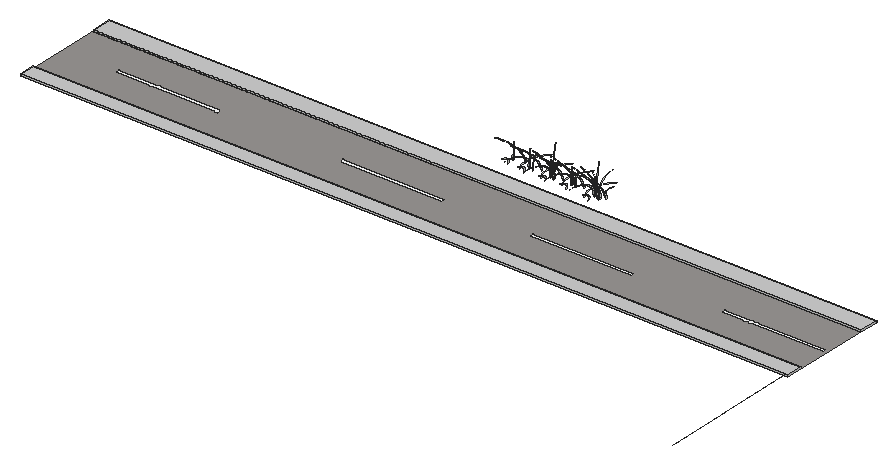
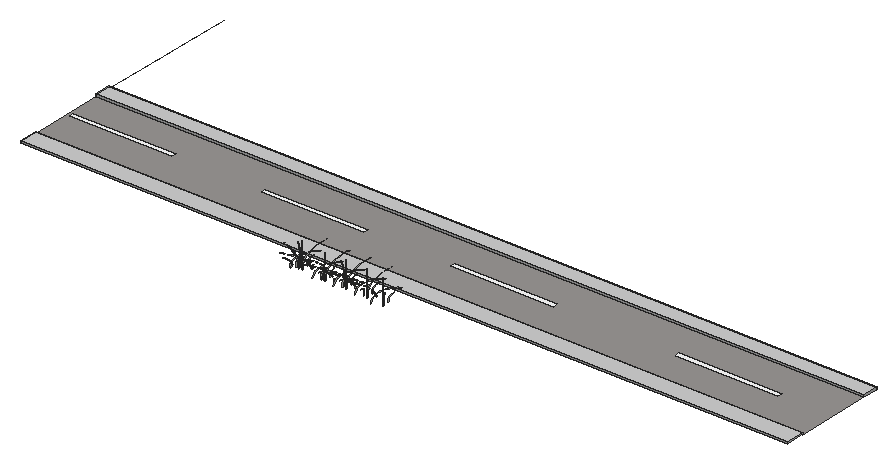
# SketchUp Ruby script. Lengths in inches.
U = 1.inch
M = Sketchup.active_model
def pt(a) = Geom::Point3d.new(a.map { |v| v * U })
def face(e, loops, mat)
  f = e.add_face(loops[0].map { |a| pt(a) })
  loops[1..].each { |l| e.add_face(l.map { |a| pt(a) }).erase! }
  f.material = f.back_material = mat if mat
  f
end
# faces: each face lists its corners as indices into pts; further lists are holes
def faces(e, pts, list, mat = nil) = list.each { |f| face(e, (f[0].is_a?(Array) ? f : [f]).map { |l| l.map { |i| pts[i] } }, mat) }
# xy, xz, yz: faces in a plane at the given z, y or x. An outline is a flat list of corners, or four numbers for a rectangle; further outlines are holes
def ring(l) = l.size == 4 ? [[l[0], l[1]], [l[2], l[1]], [l[2], l[3]], [l[0], l[3]]] : l.each_slice(2).to_a
def flat(e, list, mat, &to3) = list.each { |f| face(e, (f[0].is_a?(Array) ? f : [f]).map { |l| ring(l).map { |u, v| to3.(u, v) } }, mat) }
def xy(e, z, list, mat = nil) = flat(e, list, mat) { |x, y| [x, y, z] }
def xz(e, y, list, mat = nil) = flat(e, list, mat) { |x, z| [x, y, z] }
def yz(e, x, list, mat = nil) = flat(e, list, mat) { |y, z| [x, y, z] }
def lines(e, pts, list) = list.each { |a, b| e.add_line(pt(pts[a]), pt(pts[b])) }
# prism: a flat outline (further loops are holes) pulled along v
def prism(e, loops, v, mat = nil)
  f = face(e, loops, mat); d = Geom::Vector3d.new(v.map { |x| x * U })
  f.pushpull(f.normal.samedirection?(d) ? d.length : -d.length)
end
def box(e, o, s, mat = nil) = prism(e, [[o, [o[0] + s[0], o[1], o[2]], [o[0] + s[0], o[1] + s[1], o[2]], [o[0], o[1] + s[1], o[2]]]], [0, 0, s[2]], mat)
def at(x, y, z, deg = 0) = Geom::Transformation.translation(pt([x, y, z])) * Geom::Transformation.rotation(ORIGIN, Z_AXIS, deg.degrees)
def axes(o, x, y, z) = Geom::Transformation.new([*x, 0, *y, 0, *z, 0, *pt(o).to_a, 1])
def part(name) = M.definitions.add(name)
# library, detail: a bought-in or finely detailed component or shape, given as its bounding box
def library(name, o, s) = part(name).tap { |d| box(d.entities, o, s) }
def detail(e, o, s) = box(e.add_group.entities, o, s)
def put(e, d, t, mat = nil) = e.add_instance(d, t).tap { |i| i.material = mat if mat }
def group(e, t, mat = nil) = e.add_group.tap { |g| g.transformation = t; g.material = mat if mat }.entities
root = M.entities
M.materials.add("[Cladding_Siding_White]").color = [207, 207, 207]
M.materials.add("[Color_000]").color = [255, 255, 255]
M.materials.add("[Concrete_Aggregate_Smoke]").color = [154, 150, 148]
c1 = part("Untitled\#1")
xy(c1.entities,0,[[0,0,18.1875,211.875]],"[Cladding_Siding_White]")
xy(c1.entities,0,[[52.26,14.82,56.57,43.13],[53.72,77.12,58.03,105.43],[54.1,129.57,58.41,157.89],[54.67,182.79,58.98,211.1]],"[Color_000]")
xy(c1.entities,0,[[[18.1875,-0.0625,89.875,211.875],[52.26,14.82,56.57,43.13],[53.72,77.12,58.03,105.43],[54.1,129.57,58.41,157.89],[54.67,182.79,58.98,211.1]]],"[Concrete_Aggregate_Smoke]")
xy(c1.entities,1.625,[[0,0,18.1875,211.875]],"[Cladding_Siding_White]")
xy(c1.entities,1.9375,[[89.875,-0.0625,105,211.9375]],"[Cladding_Siding_White]")
xz(c1.entities,-0.0625,[[89.875,0,105,1.9375]],"[Cladding_Siding_White]")
xz(c1.entities,0,[[0,0,18.1875,1.625]],"[Cladding_Siding_White]")
xz(c1.entities,211.875,[[0,0,18.1875,1.625]],"[Cladding_Siding_White]")
xz(c1.entities,211.9375,[[89.875,0,105,1.9375]],"[Cladding_Siding_White]")
yz(c1.entities,0,[[0,0,211.875,1.625]],"[Cladding_Siding_White]")
yz(c1.entities,18.1875,[[0,0,211.875,1.625]],"[Cladding_Siding_White]")
yz(c1.entities,89.875,[[-0.0625,0,211.875,1.9375],[211.875,0,211.9375,1.9375]],"[Cladding_Siding_White]")
yz(c1.entities,105,[[-0.0625,0,211.9375,1.9375]],"[Cladding_Siding_White]")
p = [[799.67,134.13,1.9375],[799.67,0,0]]
lines(root,p,[[0,1]])
put(root,c1,axes([75.64,239.13,0],[0,-1,0],[3.42659,0,0],[0,0,1]))
g1 = group(root,at(519.48,258.51,0))
p = [[-0.1,-0.92,0],[-0.05,-0.41,0],[0,0,2.0625],[-0.02,-0.17,4.13],[-0.1,-0.9,6.16],[-0.24,-2.1875,8.1],
  [-0.44,-3.99,9.91],[-0.69,-6.27,11.52],[-0.99,-8.97,12.92],[-1.33,-12.02,14.05],[-1.69,-15.34,14.9],[-2.08,-18.86,15.45],
  [-2.48,-22.49,15.67],[-2.88,-26.13,15.5625],[-2.49,-22.56,15.58],[-2.1,-19.02,15.29],[-1.72,-15.6,14.71],[-1.37,-12.38,13.83],
  [-1.04,-9.43,12.68],[-0.75,-6.81,11.3],[-0.51,-4.6,9.7],[-0.3125,-2.84,7.9375],[-0.17,-1.5625,6.04],[-0.09,-0.81,4.05],
  [-0.07,-0.59,2.02]]
faces(g1,p,[[0,1,2,3,4,5,6,7,8,9,10,11,12,13,14,15,16,17,18,19,20,21,22,23,24]])
g2 = group(root,at(519.48,258.51,0))
p = [[-0.1,-0.92,0],[-0.05,-0.41,0],[0,0,2.0625],[-0.02,-0.17,4.13],[-0.1,-0.9,6.16],[-0.24,-2.1875,8.1],
  [-0.44,-3.99,9.91],[-0.69,-6.27,11.52],[-0.99,-8.97,12.92],[-1.33,-12.02,14.05],[-1.69,-15.34,14.9],[-2.08,-18.86,15.45],
  [-2.48,-22.49,15.67],[-2.88,-26.13,15.5625],[-2.49,-22.56,15.58],[-2.1,-19.02,15.29],[-1.72,-15.6,14.71],[-1.37,-12.38,13.83],
  [-1.04,-9.43,12.68],[-0.75,-6.81,11.3],[-0.51,-4.6,9.7],[-0.3125,-2.84,7.9375],[-0.17,-1.5625,6.04],[-0.09,-0.81,4.05],
  [-0.07,-0.59,2.02]]
faces(g2,p,[[0,1,2,3,4,5,6,7,8,9,10,11,12,13,14,15,16,17,18,19,20,21,22,23,24]])
g3 = group(root,at(476.43,260.84,0))
p = [[-0.1,-0.92,0],[-0.05,-0.41,0],[0,0,2.0625],[-0.02,-0.17,4.13],[-0.1,-0.9,6.16],[-0.24,-2.1875,8.1],
  [-0.44,-3.99,9.91],[-0.69,-6.27,11.52],[-0.99,-8.97,12.92],[-1.33,-12.02,14.05],[-1.69,-15.34,14.9],[-2.08,-18.86,15.45],
  [-2.48,-22.49,15.67],[-2.88,-26.13,15.5625],[-2.49,-22.56,15.58],[-2.1,-19.02,15.29],[-1.72,-15.6,14.71],[-1.37,-12.38,13.83],
  [-1.04,-9.43,12.68],[-0.75,-6.81,11.3],[-0.51,-4.6,9.7],[-0.3125,-2.84,7.9375],[-0.17,-1.5625,6.04],[-0.09,-0.81,4.05],
  [-0.07,-0.59,2.02]]
faces(g3,p,[[0,1,2,3,4,5,6,7,8,9,10,11,12,13,14,15,16,17,18,19,20,21,22,23,24]])
g4 = group(root,at(476.43,260.84,0))
p = [[-0.1,-0.92,0],[-0.05,-0.41,0],[0,0,2.0625],[-0.02,-0.17,4.13],[-0.1,-0.9,6.16],[-0.24,-2.1875,8.1],
  [-0.44,-3.99,9.91],[-0.69,-6.27,11.52],[-0.99,-8.97,12.92],[-1.33,-12.02,14.05],[-1.69,-15.34,14.9],[-2.08,-18.86,15.45],
  [-2.48,-22.49,15.67],[-2.88,-26.13,15.5625],[-2.49,-22.56,15.58],[-2.1,-19.02,15.29],[-1.72,-15.6,14.71],[-1.37,-12.38,13.83],
  [-1.04,-9.43,12.68],[-0.75,-6.81,11.3],[-0.51,-4.6,9.7],[-0.3125,-2.84,7.9375],[-0.17,-1.5625,6.04],[-0.09,-0.81,4.05],
  [-0.07,-0.59,2.02]]
faces(g4,p,[[0,1,2,3,4,5,6,7,8,9,10,11,12,13,14,15,16,17,18,19,20,21,22,23,24]])
g5 = group(root,at(520.28,251.6,0))
p = [[-0.91,-7.12,6.7],[-0.75,-5.82,6.27],[-0.6,-4.64,5.81],[-0.46,-3.6,5.31],[-0.35,-2.71,4.77],[-0.25,-1.97,4.21],
  [-0.18,-1.39,3.63],[-0.125,-0.98,3.03],[-0.09,-0.74,2.43],[-0.09,-0.67,1.8125],[-0.1,-0.77,1.2],[-0.13,-1.05,0.59],
  [-0.19,-1.49,0],[-0.12,-0.92,0],[-0.05,-0.42,0.6],[-0.01,-0.11,1.22],[0,0,1.84],[-0.01,-0.08,2.47],
  [-0.04,-0.35,3.09],[-0.1,-0.81,3.69],[-0.1875,-1.45,4.28],[-0.29,-2.27,4.84],[-0.42,-3.26,5.37],[-0.57,-4.41,5.86],
  [-0.73,-5.7,6.3]]
faces(g5,p,[[0,1,2,3,4,5,6,7,8,9,10,11,12,13,14,15,16,17,18,19,20,21,22,23,24]])
g6 = group(root,at(495.91,261.57,0))
p = [[-0.1,-0.92,0],[-0.05,-0.41,0],[0,0,2.0625],[-0.02,-0.17,4.13],[-0.1,-0.9,6.16],[-0.24,-2.1875,8.1],
  [-0.44,-3.99,9.91],[-0.69,-6.27,11.52],[-0.99,-8.97,12.92],[-1.33,-12.02,14.05],[-1.69,-15.34,14.9],[-2.08,-18.86,15.45],
  [-2.48,-22.49,15.67],[-2.88,-26.13,15.5625],[-2.49,-22.56,15.58],[-2.1,-19.02,15.29],[-1.72,-15.6,14.71],[-1.37,-12.38,13.83],
  [-1.04,-9.43,12.68],[-0.75,-6.81,11.3],[-0.51,-4.6,9.7],[-0.3125,-2.84,7.9375],[-0.17,-1.5625,6.04],[-0.09,-0.81,4.05],
  [-0.07,-0.59,2.02]]
faces(g6,p,[[0,1,2,3,4,5,6,7,8,9,10,11,12,13,14,15,16,17,18,19,20,21,22,23,24]])
g7 = group(root,at(495.91,261.57,0))
p = [[-0.1,-0.92,0],[-0.05,-0.41,0],[0,0,2.0625],[-0.02,-0.17,4.13],[-0.1,-0.9,6.16],[-0.24,-2.1875,8.1],
  [-0.44,-3.99,9.91],[-0.69,-6.27,11.52],[-0.99,-8.97,12.92],[-1.33,-12.02,14.05],[-1.69,-15.34,14.9],[-2.08,-18.86,15.45],
  [-2.48,-22.49,15.67],[-2.88,-26.13,15.5625],[-2.49,-22.56,15.58],[-2.1,-19.02,15.29],[-1.72,-15.6,14.71],[-1.37,-12.38,13.83],
  [-1.04,-9.43,12.68],[-0.75,-6.81,11.3],[-0.51,-4.6,9.7],[-0.3125,-2.84,7.9375],[-0.17,-1.5625,6.04],[-0.09,-0.81,4.05],
  [-0.07,-0.59,2.02]]
faces(g7,p,[[0,1,2,3,4,5,6,7,8,9,10,11,12,13,14,15,16,17,18,19,20,21,22,23,24]])
g8 = group(root,at(455.77,261.59,0))
p = [[-0.1,-0.92,0],[-0.05,-0.41,0],[0,0,2.0625],[-0.02,-0.17,4.13],[-0.1,-0.9,6.16],[-0.24,-2.1875,8.1],
  [-0.44,-3.99,9.91],[-0.69,-6.27,11.52],[-0.99,-8.97,12.92],[-1.33,-12.02,14.05],[-1.69,-15.34,14.9],[-2.08,-18.86,15.45],
  [-2.48,-22.49,15.67],[-2.88,-26.13,15.5625],[-2.49,-22.56,15.58],[-2.1,-19.02,15.29],[-1.72,-15.6,14.71],[-1.37,-12.38,13.83],
  [-1.04,-9.43,12.68],[-0.75,-6.81,11.3],[-0.51,-4.6,9.7],[-0.3125,-2.84,7.9375],[-0.17,-1.5625,6.04],[-0.09,-0.81,4.05],
  [-0.07,-0.59,2.02]]
faces(g8,p,[[0,1,2,3,4,5,6,7,8,9,10,11,12,13,14,15,16,17,18,19,20,21,22,23,24]])
g9 = group(root,at(455.77,261.59,0))
p = [[-0.1,-0.92,0],[-0.05,-0.41,0],[0,0,2.0625],[-0.02,-0.17,4.13],[-0.1,-0.9,6.16],[-0.24,-2.1875,8.1],
  [-0.44,-3.99,9.91],[-0.69,-6.27,11.52],[-0.99,-8.97,12.92],[-1.33,-12.02,14.05],[-1.69,-15.34,14.9],[-2.08,-18.86,15.45],
  [-2.48,-22.49,15.67],[-2.88,-26.13,15.5625],[-2.49,-22.56,15.58],[-2.1,-19.02,15.29],[-1.72,-15.6,14.71],[-1.37,-12.38,13.83],
  [-1.04,-9.43,12.68],[-0.75,-6.81,11.3],[-0.51,-4.6,9.7],[-0.3125,-2.84,7.9375],[-0.17,-1.5625,6.04],[-0.09,-0.81,4.05],
  [-0.07,-0.59,2.02]]
faces(g9,p,[[0,1,2,3,4,5,6,7,8,9,10,11,12,13,14,15,16,17,18,19,20,21,22,23,24]])
g10 = group(root,at(477.23,253.93,0))
p = [[-0.91,-7.12,6.7],[-0.75,-5.82,6.27],[-0.6,-4.64,5.81],[-0.46,-3.6,5.31],[-0.35,-2.71,4.77],[-0.25,-1.97,4.21],
  [-0.18,-1.39,3.63],[-0.125,-0.98,3.03],[-0.09,-0.74,2.43],[-0.09,-0.67,1.8125],[-0.1,-0.77,1.2],[-0.13,-1.05,0.59],
  [-0.19,-1.49,0],[-0.12,-0.92,0],[-0.05,-0.42,0.6],[-0.01,-0.11,1.22],[0,0,1.84],[-0.01,-0.08,2.47],
  [-0.04,-0.35,3.09],[-0.1,-0.81,3.69],[-0.1875,-1.45,4.28],[-0.29,-2.27,4.84],[-0.42,-3.26,5.37],[-0.57,-4.41,5.86],
  [-0.73,-5.7,6.3]]
faces(g10,p,[[0,1,2,3,4,5,6,7,8,9,10,11,12,13,14,15,16,17,18,19,20,21,22,23,24]])
g11 = group(root,at(496.71,254.67,0))
p = [[-0.91,-7.12,6.7],[-0.75,-5.82,6.27],[-0.6,-4.64,5.81],[-0.46,-3.6,5.31],[-0.35,-2.71,4.77],[-0.25,-1.97,4.21],
  [-0.18,-1.39,3.63],[-0.125,-0.98,3.03],[-0.09,-0.74,2.43],[-0.09,-0.67,1.8125],[-0.1,-0.77,1.2],[-0.13,-1.05,0.59],
  [-0.19,-1.49,0],[-0.12,-0.92,0],[-0.05,-0.42,0.6],[-0.01,-0.11,1.22],[0,0,1.84],[-0.01,-0.08,2.47],
  [-0.04,-0.35,3.09],[-0.1,-0.81,3.69],[-0.1875,-1.45,4.28],[-0.29,-2.27,4.84],[-0.42,-3.26,5.37],[-0.57,-4.41,5.86],
  [-0.73,-5.7,6.3]]
faces(g11,p,[[0,1,2,3,4,5,6,7,8,9,10,11,12,13,14,15,16,17,18,19,20,21,22,23,24]])
g12 = group(root,at(456.58,254.68,0))
p = [[-0.91,-7.12,6.7],[-0.75,-5.82,6.27],[-0.6,-4.64,5.81],[-0.46,-3.6,5.31],[-0.35,-2.71,4.77],[-0.25,-1.97,4.21],
  [-0.18,-1.39,3.63],[-0.125,-0.98,3.03],[-0.09,-0.74,2.43],[-0.09,-0.67,1.8125],[-0.1,-0.77,1.2],[-0.13,-1.05,0.59],
  [-0.19,-1.49,0],[-0.12,-0.92,0],[-0.05,-0.42,0.6],[-0.01,-0.11,1.22],[0,0,1.84],[-0.01,-0.08,2.47],
  [-0.04,-0.35,3.09],[-0.1,-0.81,3.69],[-0.1875,-1.45,4.28],[-0.29,-2.27,4.84],[-0.42,-3.26,5.37],[-0.57,-4.41,5.86],
  [-0.73,-5.7,6.3]]
faces(g12,p,[[0,1,2,3,4,5,6,7,8,9,10,11,12,13,14,15,16,17,18,19,20,21,22,23,24]])
g13 = group(root,at(439.26,257.34,0))
p = [[-0.91,-7.12,6.7],[-0.75,-5.82,6.27],[-0.6,-4.64,5.81],[-0.46,-3.6,5.31],[-0.35,-2.71,4.77],[-0.25,-1.97,4.21],
  [-0.18,-1.39,3.63],[-0.125,-0.98,3.03],[-0.09,-0.74,2.43],[-0.09,-0.67,1.8125],[-0.1,-0.77,1.2],[-0.13,-1.05,0.59],
  [-0.19,-1.49,0],[-0.12,-0.92,0],[-0.05,-0.42,0.6],[-0.01,-0.11,1.22],[0,0,1.84],[-0.01,-0.08,2.47],
  [-0.04,-0.35,3.09],[-0.1,-0.81,3.69],[-0.1875,-1.45,4.28],[-0.29,-2.27,4.84],[-0.42,-3.26,5.37],[-0.57,-4.41,5.86],
  [-0.73,-5.7,6.3]]
faces(g13,p,[[0,1,2,3,4,5,6,7,8,9,10,11,12,13,14,15,16,17,18,19,20,21,22,23,24]])
g14 = group(root,at(519.85,258.23,0))
p = [[0.57,-0.76,0],[0.25,-0.34,1.67],[0.0625,-0.09,3.36],[0,0,5.0625],[0.0625,-0.08,6.76],[0.25,-0.33,8.45],
  [0.5625,-0.75,10.12],[1,-1.34,11.77],[1.56,-2.08,13.4],[2.23,-2.99,14.98],[3.03,-4.05,16.53],[3.93,-5.26,18.02],
  [4.95,-6.62,19.46],[3.99,-5.34,18],[3.14,-4.2,16.49],[2.39,-3.19,14.9375],[1.74,-2.33,13.35],[1.2,-1.61,11.73],
  [0.77,-1.03,10.08],[0.46,-0.61,8.42],[0.25,-0.34,6.74],[0.16,-0.21,5.05],[0.18,-0.24,3.36],[0.32,-0.43,1.68]]
faces(g14,p,[[0,1,2,3,4,5,6,7,8,9,10,11,12,13,14,15,16,17,18,19,20,21,22,23]])
g15 = group(root,at(518.23,258.88,0))
p = [[5.52,-7.72,6.7],[4.47,-6.25,6.27],[3.52,-4.92,5.81],[2.68,-3.75,5.31],[1.96,-2.74,4.77],[1.37,-1.91,4.21],
  [0.9,-1.26,3.63],[0.57,-0.79,3.03],[0.37,-0.52,2.43],[0.31,-0.44,1.8125],[0.4,-0.56,1.2],[0.62,-0.87,0.59],
  [0.98,-1.37,0],[0.74,-1.03,0],[0.33,-0.46,0.59],[0.07,-0.1,1.19],[-0.04,0.05,1.81],[0.01,-0.02,2.43],
  [0.21,-0.3,3.04],[0.5625,-0.79,3.65],[1.0625,-1.49,4.23],[1.7,-2.38,4.8],[2.48,-3.47,5.33],[3.38,-4.73,5.83],
  [4.4,-6.15,6.29]]
faces(g15,p,[[0,1,2,3,4,5,6,7,8,9,10,11,12,13,14,15,16,17,18,19,20,21,22,23,24]])
g16 = group(root,at(529.54,260.45,0))
p = [[-19.18,-7.98,16.73],[-22.08,-9.1875,17.17],[-19.27,-8.02,16.64],[-16.57,-6.9,15.9],[-13.98,-5.82,14.96],[-11.56,-4.8125,13.84],
  [-9.32,-3.88,12.54],[-7.28,-3.03,11.08],[-5.47,-2.28,9.48],[-3.92,-1.63,7.76],[-2.63,-1.09,5.92],[-1.625,-0.68,4.01],
  [-0.91,-0.38,2.02],[-0.5,-0.21,0],[0,0,0],[-0.34,-0.14,2.07],[-1.01,-0.42,4.1],[-1.99,-0.83,6.07],
  [-3.29,-1.37,7.94],[-4.88,-2.03,9.7],[-6.74,-2.81,11.33],[-8.85,-3.68,12.79],[-11.18,-4.65,14.08],[-13.7,-5.7,15.17],
  [-16.375,-6.82,16.0625]]
faces(g16,p,[[0,1,2,3,4,5,6,7,8,9,10,11,12,13,14,15,16,17,18,19,20,21,22,23,24]])
g17 = group(root,at(476.8,260.56,0))
p = [[0.57,-0.76,0],[0.25,-0.34,1.67],[0.0625,-0.09,3.36],[0,0,5.0625],[0.0625,-0.08,6.76],[0.25,-0.33,8.45],
  [0.5625,-0.75,10.12],[1,-1.34,11.77],[1.56,-2.08,13.4],[2.23,-2.99,14.98],[3.03,-4.05,16.53],[3.93,-5.26,18.02],
  [4.95,-6.62,19.46],[3.99,-5.34,18],[3.14,-4.2,16.49],[2.39,-3.19,14.9375],[1.74,-2.33,13.35],[1.2,-1.61,11.73],
  [0.77,-1.03,10.08],[0.46,-0.61,8.42],[0.25,-0.34,6.74],[0.16,-0.21,5.05],[0.18,-0.24,3.36],[0.32,-0.43,1.68]]
faces(g17,p,[[0,1,2,3,4,5,6,7,8,9,10,11,12,13,14,15,16,17,18,19,20,21,22,23]])
g18 = group(root,at(475.18,261.21,0))
p = [[5.52,-7.72,6.7],[4.47,-6.25,6.27],[3.52,-4.92,5.81],[2.68,-3.75,5.31],[1.96,-2.74,4.77],[1.37,-1.91,4.21],
  [0.9,-1.26,3.63],[0.57,-0.79,3.03],[0.37,-0.52,2.43],[0.31,-0.44,1.8125],[0.4,-0.56,1.2],[0.62,-0.87,0.59],
  [0.98,-1.37,0],[0.74,-1.03,0],[0.33,-0.46,0.59],[0.07,-0.1,1.19],[-0.04,0.05,1.81],[0.01,-0.02,2.43],
  [0.21,-0.3,3.04],[0.5625,-0.79,3.65],[1.0625,-1.49,4.23],[1.7,-2.38,4.8],[2.48,-3.47,5.33],[3.38,-4.73,5.83],
  [4.4,-6.15,6.29]]
faces(g18,p,[[0,1,2,3,4,5,6,7,8,9,10,11,12,13,14,15,16,17,18,19,20,21,22,23,24]])
g19 = group(root,at(496.27,261.29,0))
p = [[0.57,-0.76,0],[0.25,-0.34,1.67],[0.0625,-0.09,3.36],[0,0,5.0625],[0.0625,-0.08,6.76],[0.25,-0.33,8.45],
  [0.5625,-0.75,10.12],[1,-1.34,11.77],[1.56,-2.08,13.4],[2.23,-2.99,14.98],[3.03,-4.05,16.53],[3.93,-5.26,18.02],
  [4.95,-6.62,19.46],[3.99,-5.34,18],[3.14,-4.2,16.49],[2.39,-3.19,14.9375],[1.74,-2.33,13.35],[1.2,-1.61,11.73],
  [0.77,-1.03,10.08],[0.46,-0.61,8.42],[0.25,-0.34,6.74],[0.16,-0.21,5.05],[0.18,-0.24,3.36],[0.32,-0.43,1.68]]
faces(g19,p,[[0,1,2,3,4,5,6,7,8,9,10,11,12,13,14,15,16,17,18,19,20,21,22,23]])
g20 = group(root,at(456.14,261.3125,0))
p = [[0.57,-0.76,0],[0.25,-0.34,1.67],[0.0625,-0.09,3.36],[0,0,5.0625],[0.0625,-0.08,6.76],[0.25,-0.33,8.45],
  [0.5625,-0.75,10.12],[1,-1.34,11.77],[1.56,-2.08,13.4],[2.23,-2.99,14.98],[3.03,-4.05,16.53],[3.93,-5.26,18.02],
  [4.95,-6.62,19.46],[3.99,-5.34,18],[3.14,-4.2,16.49],[2.39,-3.19,14.9375],[1.74,-2.33,13.35],[1.2,-1.61,11.73],
  [0.77,-1.03,10.08],[0.46,-0.61,8.42],[0.25,-0.34,6.74],[0.16,-0.21,5.05],[0.18,-0.24,3.36],[0.32,-0.43,1.68]]
faces(g20,p,[[0,1,2,3,4,5,6,7,8,9,10,11,12,13,14,15,16,17,18,19,20,21,22,23]])
g21 = group(root,at(494.65,261.94,0))
p = [[5.52,-7.72,6.7],[4.47,-6.25,6.27],[3.52,-4.92,5.81],[2.68,-3.75,5.31],[1.96,-2.74,4.77],[1.37,-1.91,4.21],
  [0.9,-1.26,3.63],[0.57,-0.79,3.03],[0.37,-0.52,2.43],[0.31,-0.44,1.8125],[0.4,-0.56,1.2],[0.62,-0.87,0.59],
  [0.98,-1.37,0],[0.74,-1.03,0],[0.33,-0.46,0.59],[0.07,-0.1,1.19],[-0.04,0.05,1.81],[0.01,-0.02,2.43],
  [0.21,-0.3,3.04],[0.5625,-0.79,3.65],[1.0625,-1.49,4.23],[1.7,-2.38,4.8],[2.48,-3.47,5.33],[3.38,-4.73,5.83],
  [4.4,-6.15,6.29]]
faces(g21,p,[[0,1,2,3,4,5,6,7,8,9,10,11,12,13,14,15,16,17,18,19,20,21,22,23,24]])
g22 = group(root,at(454.52,261.96,0))
p = [[5.52,-7.72,6.7],[4.47,-6.25,6.27],[3.52,-4.92,5.81],[2.68,-3.75,5.31],[1.96,-2.74,4.77],[1.37,-1.91,4.21],
  [0.9,-1.26,3.63],[0.57,-0.79,3.03],[0.37,-0.52,2.43],[0.31,-0.44,1.8125],[0.4,-0.56,1.2],[0.62,-0.87,0.59],
  [0.98,-1.37,0],[0.74,-1.03,0],[0.33,-0.46,0.59],[0.07,-0.1,1.19],[-0.04,0.05,1.81],[0.01,-0.02,2.43],
  [0.21,-0.3,3.04],[0.5625,-0.79,3.65],[1.0625,-1.49,4.23],[1.7,-2.38,4.8],[2.48,-3.47,5.33],[3.38,-4.73,5.83],
  [4.4,-6.15,6.29]]
faces(g22,p,[[0,1,2,3,4,5,6,7,8,9,10,11,12,13,14,15,16,17,18,19,20,21,22,23,24]])
g23 = group(root,at(486.49,262.78,0))
p = [[-19.18,-7.98,16.73],[-22.08,-9.1875,17.17],[-19.27,-8.02,16.64],[-16.57,-6.9,15.9],[-13.98,-5.82,14.96],[-11.56,-4.8125,13.84],
  [-9.32,-3.88,12.54],[-7.28,-3.03,11.08],[-5.47,-2.28,9.48],[-3.92,-1.63,7.76],[-2.63,-1.09,5.92],[-1.625,-0.68,4.01],
  [-0.91,-0.38,2.02],[-0.5,-0.21,0],[0,0,0],[-0.34,-0.14,2.07],[-1.01,-0.42,4.1],[-1.99,-0.83,6.07],
  [-3.29,-1.37,7.94],[-4.88,-2.03,9.7],[-6.74,-2.81,11.33],[-8.85,-3.68,12.79],[-11.18,-4.65,14.08],[-13.7,-5.7,15.17],
  [-16.375,-6.82,16.0625]]
faces(g23,p,[[0,1,2,3,4,5,6,7,8,9,10,11,12,13,14,15,16,17,18,19,20,21,22,23,24]])
g24 = group(root,at(505.97,263.51,0))
p = [[-19.18,-7.98,16.73],[-22.08,-9.1875,17.17],[-19.27,-8.02,16.64],[-16.57,-6.9,15.9],[-13.98,-5.82,14.96],[-11.56,-4.8125,13.84],
  [-9.32,-3.88,12.54],[-7.28,-3.03,11.08],[-5.47,-2.28,9.48],[-3.92,-1.63,7.76],[-2.63,-1.09,5.92],[-1.625,-0.68,4.01],
  [-0.91,-0.38,2.02],[-0.5,-0.21,0],[0,0,0],[-0.34,-0.14,2.07],[-1.01,-0.42,4.1],[-1.99,-0.83,6.07],
  [-3.29,-1.37,7.94],[-4.88,-2.03,9.7],[-6.74,-2.81,11.33],[-8.85,-3.68,12.79],[-11.18,-4.65,14.08],[-13.7,-5.7,15.17],
  [-16.375,-6.82,16.0625]]
faces(g24,p,[[0,1,2,3,4,5,6,7,8,9,10,11,12,13,14,15,16,17,18,19,20,21,22,23,24]])
g25 = group(root,at(465.83,263.53,0))
p = [[-19.18,-7.98,16.73],[-22.08,-9.1875,17.17],[-19.27,-8.02,16.64],[-16.57,-6.9,15.9],[-13.98,-5.82,14.96],[-11.56,-4.8125,13.84],
  [-9.32,-3.88,12.54],[-7.28,-3.03,11.08],[-5.47,-2.28,9.48],[-3.92,-1.63,7.76],[-2.63,-1.09,5.92],[-1.625,-0.68,4.01],
  [-0.91,-0.38,2.02],[-0.5,-0.21,0],[0,0,0],[-0.34,-0.14,2.07],[-1.01,-0.42,4.1],[-1.99,-0.83,6.07],
  [-3.29,-1.37,7.94],[-4.88,-2.03,9.7],[-6.74,-2.81,11.33],[-8.85,-3.68,12.79],[-11.18,-4.65,14.08],[-13.7,-5.7,15.17],
  [-16.375,-6.82,16.0625]]
faces(g25,p,[[0,1,2,3,4,5,6,7,8,9,10,11,12,13,14,15,16,17,18,19,20,21,22,23,24]])
g26 = group(root,at(514.09,252.98,0))
p = [[17.17,11.7,12.375],[19.76,13.47,12.7],[17.25,11.76,12.31],[14.83,10.11,11.76],[12.52,8.53,11.07],[10.35,7.05,10.23],
  [8.34,5.68,9.27],[6.52,4.44,8.2],[4.9,3.34,7.01],[3.51,2.39,5.74],[2.35,1.6,4.38],[1.45,0.99,2.96],
  [0.82,0.56,1.5],[0.45,0.3,0],[0,0,0],[0.3,0.21,1.53],[0.9,0.61,3.03],[1.78,1.22,4.49],
  [2.95,2.01,5.875],[4.37,2.98,7.18],[6.03,4.11,8.375],[7.92,5.4,9.46],[10,6.82,10.41],[12.26,8.36,11.22],
  [14.66,9.99,11.88]]
faces(g26,p,[[0,1,2,3,4,5,6,7,8,9,10,11,12,13,14,15,16,17,18,19,20,21,22,23,24]])
g27 = group(root,at(524.29,255.51,0))
p = [[-3.85,8.68,9.0625],[-3.11,7.03,8.49],[-2.45,5.54,7.85],[-1.87,4.22,7.18],[-1.37,3.08,6.45],[-0.95,2.15,5.7],
  [-0.625,1.41,4.91],[-0.39,0.89,4.1],[-0.26,0.58,3.28],[-0.22,0.49,2.45],[-0.28,0.625,1.625],[-0.43,0.97,0.8],
  [-0.68,1.54,0],[-0.52,1.16,0],[-0.23,0.52,0.8],[-0.05,0.11,1.61],[0.02,-0.06,2.45],[-0.01,0.02,3.28],
  [-0.15,0.33,4.11],[-0.39,0.89,4.93],[-0.74,1.67,5.72],[-1.1875,2.68,6.49],[-1.73,3.9,7.21],[-2.35,5.3125,7.88],
  [-3.0625,6.91,8.5]]
faces(g27,p,[[0,1,2,3,4,5,6,7,8,9,10,11,12,13,14,15,16,17,18,19,20,21,22,23,24]])
g28 = group(root,at(523.72,257.57,0))
p = [[-0.98,0.17,0],[-0.43,0.08,0],[0,0,1.75],[-0.18,0.03,3.51],[-0.96,0.17,5.24],[-2.32,0.41,6.89],
  [-4.24,0.76,8.42],[-6.67,1.1875,9.8],[-9.54,1.7,10.98],[-12.78,2.28,11.95],[-16.32,2.91,12.67],[-20.06,3.57,13.13],
  [-23.91,4.26,13.32],[-27.78,4.95,13.23],[-23.98,4.27,13.25],[-20.22,3.6,13],[-16.59,2.96,12.5],[-13.16,2.34,11.75],
  [-10.02,1.79,10.78],[-7.25,1.29,9.6],[-4.89,0.87,8.25],[-3.02,0.54,6.75],[-1.66,0.3,5.13],[-0.86,0.15,3.44],
  [-0.63,0.11,1.72]]
faces(g28,p,[[0,1,2,3,4,5,6,7,8,9,10,11,12,13,14,15,16,17,18,19,20,21,22,23,24]])
g29 = group(root,at(523.72,257.57,0))
p = [[-0.98,0.17,0],[-0.43,0.08,0],[0,0,1.75],[-0.18,0.03,3.51],[-0.96,0.17,5.24],[-2.32,0.41,6.89],
  [-4.24,0.76,8.42],[-6.67,1.1875,9.8],[-9.54,1.7,10.98],[-12.78,2.28,11.95],[-16.32,2.91,12.67],[-20.06,3.57,13.13],
  [-23.91,4.26,13.32],[-27.78,4.95,13.23],[-23.98,4.27,13.25],[-20.22,3.6,13],[-16.59,2.96,12.5],[-13.16,2.34,11.75],
  [-10.02,1.79,10.78],[-7.25,1.29,9.6],[-4.89,0.87,8.25],[-3.02,0.54,6.75],[-1.66,0.3,5.13],[-0.86,0.15,3.44],
  [-0.63,0.11,1.72]]
faces(g29,p,[[0,1,2,3,4,5,6,7,8,9,10,11,12,13,14,15,16,17,18,19,20,21,22,23,24]])
g30 = group(root,at(522.84,256.47,0))
p = [[-0.4,0.86,0],[-0.18,0.38,2.26],[-0.05,0.1,4.55],[0,0,6.84],[-0.04,0.09,9.14],[-0.18,0.38,11.42],
  [-0.4,0.85,13.6875],[-0.71,1.51,15.92],[-1.1,2.36,18.12],[-1.58,3.38,20.26],[-2.14,4.58,22.35],[-2.79,5.95,24.37],
  [-3.51,7.48,26.3125],[-2.83,6.04,24.34],[-2.22,4.75,22.3],[-1.69,3.61,20.2],[-1.23,2.63,18.05],[-0.85,1.82,15.86],
  [-0.55,1.17,13.64],[-0.32,0.6875,11.38],[-0.18,0.38,9.11],[-0.11,0.24,6.83],[-0.13,0.28,4.54],[-0.23,0.48,2.27]]
faces(g30,p,[[0,1,2,3,4,5,6,7,8,9,10,11,12,13,14,15,16,17,18,19,20,21,22,23]])
g31 = group(root,at(438.83,263.97,0))
p = [[0.57,-0.76,0],[0.25,-0.34,1.67],[0.0625,-0.09,3.36],[0,0,5.0625],[0.0625,-0.08,6.76],[0.25,-0.33,8.45],
  [0.5625,-0.75,10.12],[1,-1.34,11.77],[1.56,-2.08,13.4],[2.23,-2.99,14.98],[3.03,-4.05,16.53],[3.93,-5.26,18.02],
  [4.95,-6.62,19.46],[3.99,-5.34,18],[3.14,-4.2,16.49],[2.39,-3.19,14.9375],[1.74,-2.33,13.35],[1.2,-1.61,11.73],
  [0.77,-1.03,10.08],[0.46,-0.61,8.42],[0.25,-0.34,6.74],[0.16,-0.21,5.05],[0.18,-0.24,3.36],[0.32,-0.43,1.68]]
faces(g31,p,[[0,1,2,3,4,5,6,7,8,9,10,11,12,13,14,15,16,17,18,19,20,21,22,23]])
g32 = group(root,at(437.21,264.61,0))
p = [[5.52,-7.72,6.7],[4.47,-6.25,6.27],[3.52,-4.92,5.81],[2.68,-3.75,5.31],[1.96,-2.74,4.77],[1.37,-1.91,4.21],
  [0.9,-1.26,3.63],[0.57,-0.79,3.03],[0.37,-0.52,2.43],[0.31,-0.44,1.8125],[0.4,-0.56,1.2],[0.62,-0.87,0.59],
  [0.98,-1.37,0],[0.74,-1.03,0],[0.33,-0.46,0.59],[0.07,-0.1,1.19],[-0.04,0.05,1.81],[0.01,-0.02,2.43],
  [0.21,-0.3,3.04],[0.5625,-0.79,3.65],[1.0625,-1.49,4.23],[1.7,-2.38,4.8],[2.48,-3.47,5.33],[3.38,-4.73,5.83],
  [4.4,-6.15,6.29]]
faces(g32,p,[[0,1,2,3,4,5,6,7,8,9,10,11,12,13,14,15,16,17,18,19,20,21,22,23,24]])
g33 = group(root,at(448.52,266.18,0))
p = [[-19.18,-7.98,16.73],[-22.08,-9.1875,17.17],[-19.27,-8.02,16.64],[-16.57,-6.9,15.9],[-13.98,-5.82,14.96],[-11.56,-4.8125,13.84],
  [-9.32,-3.88,12.54],[-7.28,-3.03,11.08],[-5.47,-2.28,9.48],[-3.92,-1.63,7.76],[-2.63,-1.09,5.92],[-1.625,-0.68,4.01],
  [-0.91,-0.38,2.02],[-0.5,-0.21,0],[0,0,0],[-0.34,-0.14,2.07],[-1.01,-0.42,4.1],[-1.99,-0.83,6.07],
  [-3.29,-1.37,7.94],[-4.88,-2.03,9.7],[-6.74,-2.81,11.33],[-8.85,-3.68,12.79],[-11.18,-4.65,14.08],[-13.7,-5.7,15.17],
  [-16.375,-6.82,16.0625]]
faces(g33,p,[[0,1,2,3,4,5,6,7,8,9,10,11,12,13,14,15,16,17,18,19,20,21,22,23,24]])
g34 = group(root,at(471.04,255.3,0))
p = [[17.17,11.7,12.375],[19.76,13.47,12.7],[17.25,11.76,12.31],[14.83,10.11,11.76],[12.52,8.53,11.07],[10.35,7.05,10.23],
  [8.34,5.68,9.27],[6.52,4.44,8.2],[4.9,3.34,7.01],[3.51,2.39,5.74],[2.35,1.6,4.38],[1.45,0.99,2.96],
  [0.82,0.56,1.5],[0.45,0.3,0],[0,0,0],[0.3,0.21,1.53],[0.9,0.61,3.03],[1.78,1.22,4.49],
  [2.95,2.01,5.875],[4.37,2.98,7.18],[6.03,4.11,8.375],[7.92,5.4,9.46],[10,6.82,10.41],[12.26,8.36,11.22],
  [14.66,9.99,11.88]]
faces(g34,p,[[0,1,2,3,4,5,6,7,8,9,10,11,12,13,14,15,16,17,18,19,20,21,22,23,24]])
g35 = group(root,at(481.25,257.83,0))
p = [[-3.85,8.68,9.0625],[-3.11,7.03,8.49],[-2.45,5.54,7.85],[-1.87,4.22,7.18],[-1.37,3.08,6.45],[-0.95,2.15,5.7],
  [-0.625,1.41,4.91],[-0.39,0.89,4.1],[-0.26,0.58,3.28],[-0.22,0.49,2.45],[-0.28,0.625,1.625],[-0.43,0.97,0.8],
  [-0.68,1.54,0],[-0.52,1.16,0],[-0.23,0.52,0.8],[-0.05,0.11,1.61],[0.02,-0.06,2.45],[-0.01,0.02,3.28],
  [-0.15,0.33,4.11],[-0.39,0.89,4.93],[-0.74,1.67,5.72],[-1.1875,2.68,6.49],[-1.73,3.9,7.21],[-2.35,5.3125,7.88],
  [-3.0625,6.91,8.5]]
faces(g35,p,[[0,1,2,3,4,5,6,7,8,9,10,11,12,13,14,15,16,17,18,19,20,21,22,23,24]])
g36 = group(root,at(480.67,259.89,0))
p = [[-0.98,0.17,0],[-0.43,0.08,0],[0,0,1.75],[-0.18,0.03,3.51],[-0.96,0.17,5.24],[-2.32,0.41,6.89],
  [-4.24,0.76,8.42],[-6.67,1.1875,9.8],[-9.54,1.7,10.98],[-12.78,2.28,11.95],[-16.32,2.91,12.67],[-20.06,3.57,13.13],
  [-23.91,4.26,13.32],[-27.78,4.95,13.23],[-23.98,4.27,13.25],[-20.22,3.6,13],[-16.59,2.96,12.5],[-13.16,2.34,11.75],
  [-10.02,1.79,10.78],[-7.25,1.29,9.6],[-4.89,0.87,8.25],[-3.02,0.54,6.75],[-1.66,0.3,5.13],[-0.86,0.15,3.44],
  [-0.63,0.11,1.72]]
faces(g36,p,[[0,1,2,3,4,5,6,7,8,9,10,11,12,13,14,15,16,17,18,19,20,21,22,23,24]])
g37 = group(root,at(480.67,259.89,0))
p = [[-0.98,0.17,0],[-0.43,0.08,0],[0,0,1.75],[-0.18,0.03,3.51],[-0.96,0.17,5.24],[-2.32,0.41,6.89],
  [-4.24,0.76,8.42],[-6.67,1.1875,9.8],[-9.54,1.7,10.98],[-12.78,2.28,11.95],[-16.32,2.91,12.67],[-20.06,3.57,13.13],
  [-23.91,4.26,13.32],[-27.78,4.95,13.23],[-23.98,4.27,13.25],[-20.22,3.6,13],[-16.59,2.96,12.5],[-13.16,2.34,11.75],
  [-10.02,1.79,10.78],[-7.25,1.29,9.6],[-4.89,0.87,8.25],[-3.02,0.54,6.75],[-1.66,0.3,5.13],[-0.86,0.15,3.44],
  [-0.63,0.11,1.72]]
faces(g37,p,[[0,1,2,3,4,5,6,7,8,9,10,11,12,13,14,15,16,17,18,19,20,21,22,23,24]])
g38 = group(root,at(525.9,256.14,0))
p = [[-0.62,0.44,0],[-0.27,0.2,0],[0,0,1.68],[-0.11,0.08,3.37],[-0.6,0.43,5.03],[-1.46,1.05,6.61],
  [-2.67,1.92,8.08],[-4.2,3.02,9.4],[-6.01,4.32,10.54],[-8.05,5.79,11.47],[-10.28,7.39,12.16],[-12.64,9.08,12.61],
  [-15.07,10.83,12.79],[-17.5,12.58,12.7],[-15.11,10.86,12.72],[-12.74,9.16,12.48],[-10.45,7.51,12],[-8.29,5.96,11.29],
  [-6.32,4.54,10.35],[-4.57,3.28,9.22],[-3.08,2.21,7.92],[-1.9,1.37,6.48],[-1.05,0.75,4.93],[-0.54,0.39,3.31],
  [-0.4,0.29,1.65]]
faces(g38,p,[[0,1,2,3,4,5,6,7,8,9,10,11,12,13,14,15,16,17,18,19,20,21,22,23,24]])
g39 = group(root,at(522.64,258.72,0))
p = [[7.51,7.51,22.54],[6.3125,6.3125,20.88],[5.21,5.21,19.16],[4.21,4.21,17.39],[3.32,3.32,15.57],[2.52,2.52,13.71],
  [1.84,1.84,11.82],[1.27,1.27,9.89],[0.81,0.81,7.94],[0.46,0.46,5.97],[0.22,0.22,3.99],[0.1,0.1,2],
  [0.1,0.1,0],[0,0,2.01],[0.04,0.04,4.01],[0.21,0.21,6.01],[0.51,0.51,8],[0.95,0.95,9.97],
  [1.51,1.51,11.91],[2.21,2.21,13.81],[3.03,3.03,15.67],[3.98,3.98,17.48],[5.04,5.04,19.23],[6.22,6.22,20.92]]
faces(g39,p,[[0,1,2,3,4,5,6,7,8,9,10,11,12,13,14,15,16,17,18,19,20,21,22,23]])
g40 = group(root,at(526.07,257.53,0))
p = [[-0.93,0.35,0],[-0.41,0.16,0],[0,0,1.75],[-0.17,0.0625,3.51],[-0.91,0.34,5.24],[-2.21,0.83,6.89],
  [-4.03,1.52,8.42],[-6.34,2.39,9.8],[-9.0625,3.42,10.98],[-12.14,4.59,11.95],[-15.5,5.86,12.67],[-19.06,7.2,13.13],
  [-22.72,8.58,13.32],[-26.4,9.97,13.23],[-22.79,8.61,13.25],[-19.22,7.26,13],[-15.76,5.96,12.5],[-12.51,4.73,11.75],
  [-9.53,3.6,10.78],[-6.89,2.6,9.6],[-4.65,1.76,8.25],[-2.87,1.08,6.75],[-1.58,0.6,5.13],[-0.82,0.31,3.44],
  [-0.6,0.23,1.72]]
faces(g40,p,[[0,1,2,3,4,5,6,7,8,9,10,11,12,13,14,15,16,17,18,19,20,21,22,23,24]])
g41 = group(root,at(479.79,258.8,0))
p = [[-0.4,0.86,0],[-0.18,0.38,2.26],[-0.05,0.1,4.55],[0,0,6.84],[-0.04,0.09,9.14],[-0.18,0.38,11.42],
  [-0.4,0.85,13.6875],[-0.71,1.51,15.92],[-1.1,2.36,18.12],[-1.58,3.38,20.26],[-2.14,4.58,22.35],[-2.79,5.95,24.37],
  [-3.51,7.48,26.3125],[-2.83,6.04,24.34],[-2.22,4.75,22.3],[-1.69,3.61,20.2],[-1.23,2.63,18.05],[-0.85,1.82,15.86],
  [-0.55,1.17,13.64],[-0.32,0.6875,11.38],[-0.18,0.38,9.11],[-0.11,0.24,6.83],[-0.13,0.28,4.54],[-0.23,0.48,2.27]]
faces(g41,p,[[0,1,2,3,4,5,6,7,8,9,10,11,12,13,14,15,16,17,18,19,20,21,22,23]])
g42 = group(root,at(490.51,256.04,0))
p = [[17.17,11.7,12.375],[19.76,13.47,12.7],[17.25,11.76,12.31],[14.83,10.11,11.76],[12.52,8.53,11.07],[10.35,7.05,10.23],
  [8.34,5.68,9.27],[6.52,4.44,8.2],[4.9,3.34,7.01],[3.51,2.39,5.74],[2.35,1.6,4.38],[1.45,0.99,2.96],
  [0.82,0.56,1.5],[0.45,0.3,0],[0,0,0],[0.3,0.21,1.53],[0.9,0.61,3.03],[1.78,1.22,4.49],
  [2.95,2.01,5.875],[4.37,2.98,7.18],[6.03,4.11,8.375],[7.92,5.4,9.46],[10,6.82,10.41],[12.26,8.36,11.22],
  [14.66,9.99,11.88]]
faces(g42,p,[[0,1,2,3,4,5,6,7,8,9,10,11,12,13,14,15,16,17,18,19,20,21,22,23,24]])
g43 = group(root,at(450.38,256.06,0))
p = [[17.17,11.7,12.375],[19.76,13.47,12.7],[17.25,11.76,12.31],[14.83,10.11,11.76],[12.52,8.53,11.07],[10.35,7.05,10.23],
  [8.34,5.68,9.27],[6.52,4.44,8.2],[4.9,3.34,7.01],[3.51,2.39,5.74],[2.35,1.6,4.38],[1.45,0.99,2.96],
  [0.82,0.56,1.5],[0.45,0.3,0],[0,0,0],[0.3,0.21,1.53],[0.9,0.61,3.03],[1.78,1.22,4.49],
  [2.95,2.01,5.875],[4.37,2.98,7.18],[6.03,4.11,8.375],[7.92,5.4,9.46],[10,6.82,10.41],[12.26,8.36,11.22],
  [14.66,9.99,11.88]]
faces(g43,p,[[0,1,2,3,4,5,6,7,8,9,10,11,12,13,14,15,16,17,18,19,20,21,22,23,24]])
g44 = group(root,at(500.72,258.57,0))
p = [[-3.85,8.68,9.0625],[-3.11,7.03,8.49],[-2.45,5.54,7.85],[-1.87,4.22,7.18],[-1.37,3.08,6.45],[-0.95,2.15,5.7],
  [-0.625,1.41,4.91],[-0.39,0.89,4.1],[-0.26,0.58,3.28],[-0.22,0.49,2.45],[-0.28,0.625,1.625],[-0.43,0.97,0.8],
  [-0.68,1.54,0],[-0.52,1.16,0],[-0.23,0.52,0.8],[-0.05,0.11,1.61],[0.02,-0.06,2.45],[-0.01,0.02,3.28],
  [-0.15,0.33,4.11],[-0.39,0.89,4.93],[-0.74,1.67,5.72],[-1.1875,2.68,6.49],[-1.73,3.9,7.21],[-2.35,5.3125,7.88],
  [-3.0625,6.91,8.5]]
faces(g44,p,[[0,1,2,3,4,5,6,7,8,9,10,11,12,13,14,15,16,17,18,19,20,21,22,23,24]])
g45 = group(root,at(460.59,258.59,0))
p = [[-3.85,8.68,9.0625],[-3.11,7.03,8.49],[-2.45,5.54,7.85],[-1.87,4.22,7.18],[-1.37,3.08,6.45],[-0.95,2.15,5.7],
  [-0.625,1.41,4.91],[-0.39,0.89,4.1],[-0.26,0.58,3.28],[-0.22,0.49,2.45],[-0.28,0.625,1.625],[-0.43,0.97,0.8],
  [-0.68,1.54,0],[-0.52,1.16,0],[-0.23,0.52,0.8],[-0.05,0.11,1.61],[0.02,-0.06,2.45],[-0.01,0.02,3.28],
  [-0.15,0.33,4.11],[-0.39,0.89,4.93],[-0.74,1.67,5.72],[-1.1875,2.68,6.49],[-1.73,3.9,7.21],[-2.35,5.3125,7.88],
  [-3.0625,6.91,8.5]]
faces(g45,p,[[0,1,2,3,4,5,6,7,8,9,10,11,12,13,14,15,16,17,18,19,20,21,22,23,24]])
g46 = group(root,at(527.1,260.44,0))
p = [[5.08,5.08,9.0625],[4.15,4.15,8.49],[3.31,3.31,7.85],[2.57,2.57,7.18],[1.93,1.93,6.45],[1.41,1.41,5.7],
  [0.99,0.99,4.91],[0.7,0.7,4.1],[0.53,0.53,3.28],[0.48,0.48,2.45],[0.55,0.55,1.625],[0.75,0.75,0.8],
  [1.0625,1.0625,0],[0.65,0.65,0],[0.3,0.3,0.81],[0.08,0.08,1.65],[0,0,2.49],[0.06,0.06,3.34],
  [0.25,0.25,4.17],[0.58,0.58,4.99],[1.04,1.04,5.79],[1.62,1.62,6.54],[2.33,2.33,7.26],[3.14,3.14,7.92],
  [4.0625,4.0625,8.52]]
faces(g46,p,[[0,1,2,3,4,5,6,7,8,9,10,11,12,13,14,15,16,17,18,19,20,21,22,23,24]])
g47 = group(root,at(500.15,260.63,0))
p = [[-0.98,0.17,0],[-0.43,0.08,0],[0,0,1.75],[-0.18,0.03,3.51],[-0.96,0.17,5.24],[-2.32,0.41,6.89],
  [-4.24,0.76,8.42],[-6.67,1.1875,9.8],[-9.54,1.7,10.98],[-12.78,2.28,11.95],[-16.32,2.91,12.67],[-20.06,3.57,13.13],
  [-23.91,4.26,13.32],[-27.78,4.95,13.23],[-23.98,4.27,13.25],[-20.22,3.6,13],[-16.59,2.96,12.5],[-13.16,2.34,11.75],
  [-10.02,1.79,10.78],[-7.25,1.29,9.6],[-4.89,0.87,8.25],[-3.02,0.54,6.75],[-1.66,0.3,5.13],[-0.86,0.15,3.44],
  [-0.63,0.11,1.72]]
faces(g47,p,[[0,1,2,3,4,5,6,7,8,9,10,11,12,13,14,15,16,17,18,19,20,21,22,23,24]])
g48 = group(root,at(500.15,260.63,0))
p = [[-0.98,0.17,0],[-0.43,0.08,0],[0,0,1.75],[-0.18,0.03,3.51],[-0.96,0.17,5.24],[-2.32,0.41,6.89],
  [-4.24,0.76,8.42],[-6.67,1.1875,9.8],[-9.54,1.7,10.98],[-12.78,2.28,11.95],[-16.32,2.91,12.67],[-20.06,3.57,13.13],
  [-23.91,4.26,13.32],[-27.78,4.95,13.23],[-23.98,4.27,13.25],[-20.22,3.6,13],[-16.59,2.96,12.5],[-13.16,2.34,11.75],
  [-10.02,1.79,10.78],[-7.25,1.29,9.6],[-4.89,0.87,8.25],[-3.02,0.54,6.75],[-1.66,0.3,5.13],[-0.86,0.15,3.44],
  [-0.63,0.11,1.72]]
faces(g48,p,[[0,1,2,3,4,5,6,7,8,9,10,11,12,13,14,15,16,17,18,19,20,21,22,23,24]])
